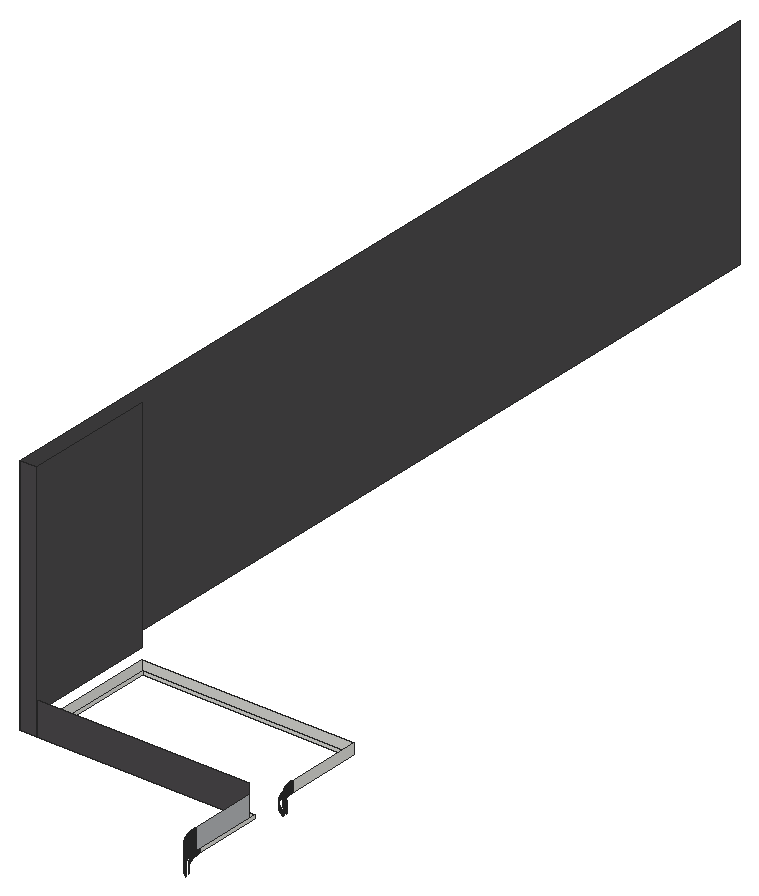
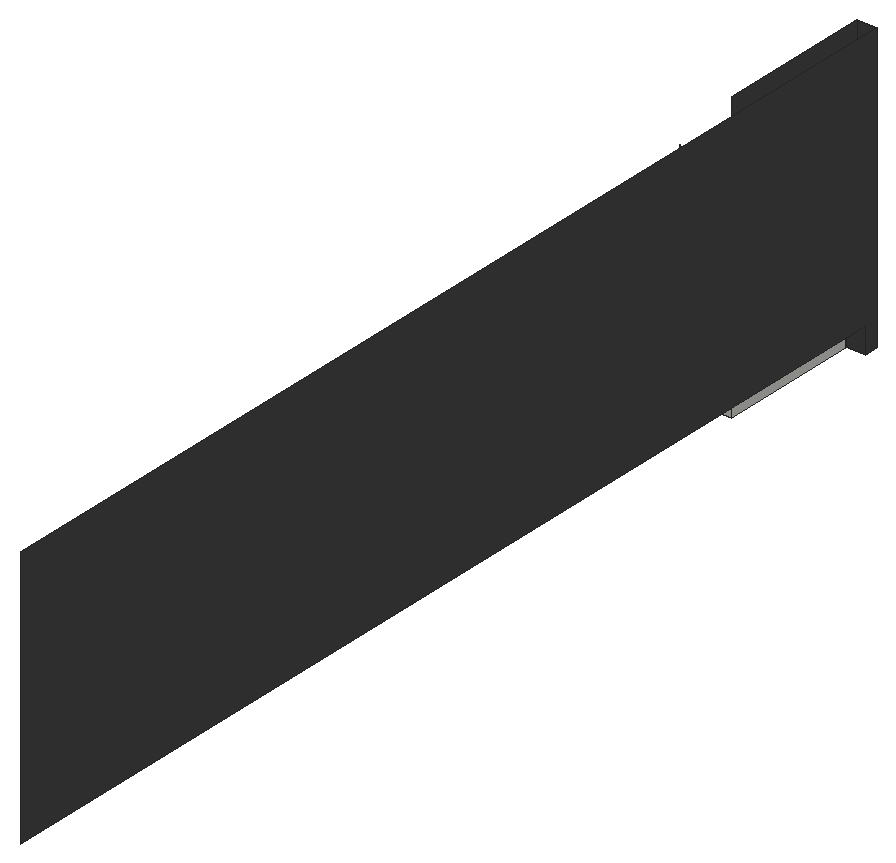
# SketchUp Ruby script. Lengths in inches.
U = 1.inch
M = Sketchup.active_model
def pt(a) = Geom::Point3d.new(a.map { |v| v * U })
def face(e, loops, mat)
  f = e.add_face(loops[0].map { |a| pt(a) })
  loops[1..].each { |l| e.add_face(l.map { |a| pt(a) }).erase! }
  f.material = f.back_material = mat if mat
  f
end
# faces: each face lists its corners as indices into pts; further lists are holes
def faces(e, pts, list, mat = nil) = list.each { |f| face(e, (f[0].is_a?(Array) ? f : [f]).map { |l| l.map { |i| pts[i] } }, mat) }
# xy, xz, yz: faces in a plane at the given z, y or x. An outline is a flat list of corners, or four numbers for a rectangle; further outlines are holes
def ring(l) = l.size == 4 ? [[l[0], l[1]], [l[2], l[1]], [l[2], l[3]], [l[0], l[3]]] : l.each_slice(2).to_a
def flat(e, list, mat, &to3) = list.each { |f| face(e, (f[0].is_a?(Array) ? f : [f]).map { |l| ring(l).map { |u, v| to3.(u, v) } }, mat) }
def xy(e, z, list, mat = nil) = flat(e, list, mat) { |x, y| [x, y, z] }
def xz(e, y, list, mat = nil) = flat(e, list, mat) { |x, z| [x, y, z] }
def yz(e, x, list, mat = nil) = flat(e, list, mat) { |y, z| [x, y, z] }
def lines(e, pts, list) = list.each { |a, b| e.add_line(pt(pts[a]), pt(pts[b])) }
# prism: a flat outline (further loops are holes) pulled along v
def prism(e, loops, v, mat = nil)
  f = face(e, loops, mat); d = Geom::Vector3d.new(v.map { |x| x * U })
  f.pushpull(f.normal.samedirection?(d) ? d.length : -d.length)
end
def box(e, o, s, mat = nil) = prism(e, [[o, [o[0] + s[0], o[1], o[2]], [o[0] + s[0], o[1] + s[1], o[2]], [o[0], o[1] + s[1], o[2]]]], [0, 0, s[2]], mat)
def at(x, y, z, deg = 0) = Geom::Transformation.translation(pt([x, y, z])) * Geom::Transformation.rotation(ORIGIN, Z_AXIS, deg.degrees)
def axes(o, x, y, z) = Geom::Transformation.new([*x, 0, *y, 0, *z, 0, *pt(o).to_a, 1])
def part(name) = M.definitions.add(name)
# library, detail: a bought-in or finely detailed component or shape, given as its bounding box
def library(name, o, s) = part(name).tap { |d| box(d.entities, o, s) }
def detail(e, o, s) = box(e.add_group.entities, o, s)
def put(e, d, t, mat = nil) = e.add_instance(d, t).tap { |i| i.material = mat if mat }
def group(e, t, mat = nil) = e.add_group.tap { |g| g.transformation = t; g.material = mat if mat }.entities
root = M.entities
M.materials.add("1423 AP 8230 BENTONITE").color = [77, 75, 77]
M.materials.add("1427 AP 686 ARMOUR-N").color = [184, 186, 189]
xy(root,114,[[9,180,18,186]],"1423 AP 8230 BENTONITE")
xy(root,114,[[9,180,18,186]],"1427 AP 686 ARMOUR-N")
xz(root,180,[[9,114,18,246],[18,114,134,132]],"1423 AP 8230 BENTONITE")
xz(root,182,[[20,114,136,116]])
xz(root,186,[[9,114,18,126]],"1423 AP 8230 BENTONITE")
xz(root,186,[[9,114,18,120]],"1427 AP 686 ARMOUR-N")
xz(root,250,[[20,114,132,116]])
xz(root,252,[[18,114,134,120]])
yz(root,9,[[180,114,180,246,672,246,672,126,186,126,186,114]],"1423 AP 8230 BENTONITE")
yz(root,18,[[180,114,180,132,186,132,186,120,252,120,252,114]])
yz(root,18,[[180,114,186,114,186,126,252,126,252,246,180,246]],"1423 AP 8230 BENTONITE")
yz(root,20,[[182,114,250,116]])
yz(root,132,[[209.76,114,209.96,116],[209.96,114,210,116],[210,114,250,116]])
yz(root,132.01,[[209.28,114,209.52,116]])
yz(root,134,[[209.78,114,209.97,120],[209.97,114,210,120],[209.97,114,210,120],[210,114,252,120]])
yz(root,134,[[143.6875,114,144,126],[144,114,180,126]],"1427 AP 686 ARMOUR-N")
yz(root,134.01,[[209.35,114,209.57,120]])
yz(root,136,[[143.71,114,144,116],[144,114,182,116]])
p = [[143.89,124.58,126],[143.64,124.77,126],[143.64,124.77,114],[143.89,124.58,114],[143.39,124.96,126],[143.39,124.96,114],
  [143.14,125.15,126],[143.14,125.15,114],[142.9,125.35,126],[142.9,125.35,114],[142.65,125.55,126],[142.65,125.55,114],
  [142.41,125.75,126],[142.41,125.75,114],[142.18,125.96,126],[142.18,125.96,114],[141.94,126.16,126],[141.94,126.16,114],
  [141.71,126.375,126],[141.71,126.375,114],[141.48,126.59,126],[141.48,126.59,114],[141.25,126.81,126],[141.25,126.81,114],
  [141.03,127.03,126],[141.03,127.03,114],[140.81,127.25,126],[140.81,127.25,114],[140.59,127.48,126],[140.59,127.48,114],
  [143.71,127.27,114],[143.49,127.46,114],[143.49,127.46,116],[143.71,127.27,116],[140.375,127.71,126],[140.375,127.71,114],
  [143.28,127.65,114],[143.28,127.65,116],[140.16,127.94,126],[140.16,127.94,114],[143.07,127.84,114],[143.07,127.84,116],
  [142.86,128.04,114],[142.86,128.04,116],[139.96,128.18,126],[139.96,128.18,114],[142.65,128.24,114],[142.65,128.24,116],
  [139.75,128.41,126],[139.75,128.41,114],[142.44,128.44,114],[142.44,128.44,116],[139.55,128.65,126],[139.55,128.65,114],
  [142.24,128.65,114],[142.24,128.65,116],[142.04,128.86,114],[142.04,128.86,116],[139.35,128.9,126],[139.35,128.9,114],
  [139.15,129.14,126],[139.15,129.14,114],[141.84,129.07,114],[141.84,129.07,116],[138.96,129.39,126],[138.96,129.39,114],
  [141.65,129.28,114],[141.65,129.28,116],[141.46,129.49,114],[141.46,129.49,116],[138.77,129.64,126],[138.77,129.64,114],
  [141.27,129.71,114],[141.27,129.71,116],[138.58,129.89,126],[138.58,129.89,114],[141.09,129.93,114],[141.09,129.93,116],
  [138.4,130.15,126],[138.4,130.15,114],[140.9,130.15,114],[140.9,130.15,116],[138.22,130.41,126],[138.22,130.41,114],
  [140.72,130.38,114],[140.72,130.38,116],[138.04,130.67,126],[138.04,130.67,114],[140.55,130.61,114],[140.55,130.61,116],
  [140.37,130.84,114],[140.37,130.84,116],[137.87,130.93,126],[137.87,130.93,114],[140.2,131.07,114],[140.2,131.07,116],
  [137.7,131.19,126],[137.7,131.19,114],[140.03,131.3,114],[140.03,131.3,116],[137.54,131.46,126],[137.54,131.46,114],
  [139.87,131.54,114],[139.87,131.54,116],[137.375,131.73,126],[137.375,131.73,114],[139.71,131.78,114],[139.71,131.78,116],
  [137.22,132,126],[137.22,132,114],[139.55,132.02,114],[139.55,132.02,116],[137.06,132.27,126],[137.06,132.27,114],
  [139.39,132.26,114],[139.39,132.26,116],[136.91,132.55,126],[136.91,132.55,114],[139.24,132.51,114],[139.24,132.51,116],
  [136.76,132.83,126],[136.76,132.83,114],[139.09,132.75,114],[139.09,132.75,116],[136.62,133.1,126],[136.62,133.1,114],
  [138.95,133,114],[138.95,133,116],[138.81,133.25,114],[138.81,133.25,116],[136.48,133.39,126],[136.48,133.39,114],
  [138.67,133.5,114],[138.67,133.5,116],[136.34,133.67,126],[136.34,133.67,114],[138.53,133.76,114],[138.53,133.76,116],
  [136.2,133.95,126],[136.2,133.95,114],[138.4,134.01,114],[138.4,134.01,116],[136.07,134.24,126],[136.07,134.24,114],
  [138.27,134.27,114],[138.27,134.27,116],[135.95,134.53,126],[135.95,134.53,114],[138.14,134.53,114],[138.14,134.53,116],
  [135.83,134.82,126],[135.83,134.82,114],[138.02,134.79,114],[138.02,134.79,116],[135.71,135.11,126],[135.71,135.11,114],
  [137.9,135.05,114],[137.9,135.05,116],[135.59,135.4,126],[135.59,135.4,114],[137.79,135.32,114],[137.79,135.32,116],
  [137.67,135.58,114],[137.67,135.58,116],[135.48,135.69,126],[135.48,135.69,114],[137.57,135.85,114],[137.57,135.85,116],
  [135.375,135.99,126],[135.375,135.99,114],[137.46,136.12,114],[137.46,136.12,116],[135.27,136.29,126],[135.27,136.29,114],
  [137.36,136.39,114],[137.36,136.39,116],[135.17,136.58,126],[135.17,136.58,114],[137.26,136.66,114],[137.26,136.66,116],
  [135.08,136.88,126],[135.08,136.88,114],[137.17,136.93,114],[137.17,136.93,116],[134.99,137.18,126],[134.99,137.18,114],
  [137.08,137.2,114],[137.08,137.2,116],[134.9,137.49,126],[134.9,137.49,114],[136.99,137.48,114],[136.99,137.48,116],
  [134.82,137.79,126],[134.82,137.79,114],[136.91,137.75,114],[136.91,137.75,116],[134.74,138.09,126],[134.74,138.09,114],
  [136.83,138.03,114],[136.83,138.03,116],[136.75,138.31,114],[136.75,138.31,116],[134.66,138.4,126],[134.66,138.4,114],
  [136.68,138.58,114],[136.68,138.58,116],[134.59,138.7,126],[134.59,138.7,114],[136.61,138.86,114],[136.61,138.86,116],
  [134.52,139.01,126],[134.52,139.01,114],[136.54,139.14,114],[136.54,139.14,116],[134.46,139.32,126],[134.46,139.32,114],
  [136.48,139.43,114],[136.48,139.43,116],[134.4,139.625,126],[134.4,139.625,114],[136.42,139.71,114],[136.42,139.71,116],
  [134.35,139.9375,126],[134.35,139.9375,114],[136.37,139.99,114],[136.37,139.99,116],[134.3,140.25,126],[134.3,140.25,114],
  [136.32,140.27,114],[136.32,140.27,116],[134.25,140.56,126],[134.25,140.56,114],[136.27,140.56,114],[136.27,140.56,116],
  [134.21,140.87,126],[134.21,140.87,114],[136.23,140.84,114],[136.23,140.84,116],[136.1875,141.13,114],[136.1875,141.13,116],
  [134.17,141.18,126],[134.17,141.18,114],[136.15,141.41,114],[136.15,141.41,116],[134.13,141.49,126],[134.13,141.49,114],
  [136.12,141.7,114],[136.12,141.7,116],[134.1,141.8,126],[134.1,141.8,114],[136.09,141.99,114],[136.09,141.99,116],
  [134.07,142.12,126],[134.07,142.12,114],[136.07,142.27,114],[136.07,142.27,116],[134.05,142.43,126],[134.05,142.43,114],
  [136.05,142.5625,114],[136.05,142.5625,116],[134.03,142.74,126],[134.03,142.74,114],[136.03,142.85,114],[136.03,142.85,116],
  [134.02,143.06,126],[134.02,143.06,114],[136.02,143.14,114],[136.02,143.14,116],[134.01,143.37,126],[134.01,143.37,114],
  [136.01,143.42,114],[136.01,143.42,116],[134,143.6875,126],[134,143.6875,114],[136,143.71,114],[136,143.71,116],
  [143.57,191.86,114],[143.79,191.76,114],[143.79,191.76,116],[143.57,191.86,116],[143.35,191.97,114],[143.35,191.97,116],
  [143.14,192.07,114],[143.14,192.07,116],[142.92,192.18,114],[142.92,192.18,116],[142.71,192.29,114],[142.71,192.29,116],
  [142.49,192.4,114],[142.49,192.4,116],[142.28,192.52,114],[142.28,192.52,116],[142.07,192.64,114],[142.07,192.64,116],
  [141.86,192.76,114],[141.86,192.76,116],[141.65,192.88,114],[141.65,192.88,116],[141.45,193.01,114],[141.45,193.01,116],
  [141.24,193.14,114],[141.24,193.14,116],[141.04,193.27,114],[141.04,193.27,116],[140.84,193.4,114],[140.84,193.4,116],
  [140.64,193.54,114],[140.64,193.54,116],[140.44,193.68,114],[140.44,193.68,116],[140.24,193.82,114],[140.24,193.82,116],
  [140.05,193.96,114],[140.05,193.96,116],[139.86,194.11,114],[139.86,194.11,116],[143.63,194.0625,120],[143.83,193.96,120],
  [143.83,193.96,114],[143.63,194.0625,114],[139.67,194.26,114],[139.67,194.26,116],[143.44,194.16,120],[143.44,194.16,114],
  [143.25,194.27,120],[143.25,194.27,114],[139.48,194.41,114],[139.48,194.41,116],[143.0625,194.375,120],[143.0625,194.375,114],
  [139.29,194.56,114],[139.29,194.56,116],[142.875,194.48,120],[142.875,194.48,114],[142.6875,194.6,120],[142.6875,194.6,114],
  [139.1,194.71,114],[139.1,194.71,116],[142.5,194.71,120],[142.5,194.71,114],[138.92,194.87,114],[138.92,194.87,116],
  [142.32,194.83,120],[142.32,194.83,114],[142.14,194.94,120],[142.14,194.94,114],[138.74,195.03,114],[138.74,195.03,116],
  [141.95,195.0625,120],[141.95,195.0625,114],[138.56,195.19,114],[138.56,195.19,116],[141.77,195.1875,120],[141.77,195.1875,114],
  [138.38,195.35,114],[138.38,195.35,116],[141.6,195.3125,120],[141.6,195.3125,114],[141.42,195.4375,120],[141.42,195.4375,114],
  [138.2,195.52,114],[138.2,195.52,116],[141.24,195.57,120],[141.24,195.57,114],[138.03,195.6875,114],[138.03,195.6875,116],
  [141.07,195.7,120],[141.07,195.7,114],[137.86,195.86,114],[137.86,195.86,116],[140.9,195.83,120],[140.9,195.83,114],
  [140.73,195.97,120],[140.73,195.97,114],[137.6875,196.03,114],[137.6875,196.03,116],[137.52,196.2,114],[137.52,196.2,116],
  [140.56,196.1,120],[140.56,196.1,114],[140.39,196.24,120],[140.39,196.24,114],[137.35,196.38,114],[137.35,196.38,116],
  [140.23,196.38,120],[140.23,196.38,114],[137.19,196.56,114],[137.19,196.56,116],[140.0625,196.53,120],[140.0625,196.53,114],
  [139.9,196.67,120],[139.9,196.67,114],[137.03,196.74,114],[137.03,196.74,116],[136.87,196.92,114],[136.87,196.92,116],
  [139.74,196.82,120],[139.74,196.82,114],[139.58,196.97,120],[139.58,196.97,114],[136.71,197.1,114],[136.71,197.1,116],
  [139.43,197.12,120],[139.43,197.12,114],[136.56,197.29,114],[136.56,197.29,116],[139.27,197.27,120],[139.27,197.27,114],
  [136.41,197.48,114],[136.41,197.48,116],[139.12,197.43,120],[139.12,197.43,114],[138.97,197.58,120],[138.97,197.58,114],
  [136.26,197.67,114],[136.26,197.67,116],[138.82,197.74,120],[138.82,197.74,114],[136.11,197.86,114],[136.11,197.86,116],
  [138.67,197.9,120],[138.67,197.9,114],[135.96,198.05,114],[135.96,198.05,116],[138.53,198.0625,120],[138.53,198.0625,114],
  [135.82,198.24,114],[135.82,198.24,116],[138.38,198.23,120],[138.38,198.23,114],[135.68,198.44,114],[135.68,198.44,116],
  [138.24,198.39,120],[138.24,198.39,114],[135.54,198.64,114],[135.54,198.64,116],[138.1,198.56,120],[138.1,198.56,114],
  [135.4,198.84,114],[135.4,198.84,116],[137.97,198.73,120],[137.97,198.73,114],[137.83,198.9,120],[137.83,198.9,114],
  [135.27,199.04,114],[135.27,199.04,116],[137.7,199.07,120],[137.7,199.07,114],[135.14,199.24,114],[135.14,199.24,116],
  [137.57,199.24,120],[137.57,199.24,114],[135.01,199.45,114],[135.01,199.45,116],[137.4375,199.42,120],[137.4375,199.42,114],
  [134.88,199.65,114],[134.88,199.65,116],[137.3125,199.6,120],[137.3125,199.6,114],[137.1875,199.77,120],[137.1875,199.77,114],
  [134.76,199.86,114],[134.76,199.86,116],[137.0625,199.95,120],[137.0625,199.95,114],[134.64,200.07,114],[134.64,200.07,116],
  [136.94,200.14,120],[136.94,200.14,114],[134.52,200.28,114],[134.52,200.28,116],[136.83,200.32,120],[136.83,200.32,114],
  [134.4,200.49,114],[134.4,200.49,116],[136.71,200.5,120],[136.71,200.5,114],[134.29,200.71,114],[134.29,200.71,116],
  [136.6,200.6875,120],[136.6,200.6875,114],[134.18,200.92,114],[134.18,200.92,116],[136.48,200.875,120],[136.48,200.875,114],
  [134.07,201.14,114],[134.07,201.14,116],[136.375,201.0625,120],[136.375,201.0625,114],[133.97,201.35,114],[133.97,201.35,116],
  [136.27,201.25,120],[136.27,201.25,114],[136.16,201.44,120],[136.16,201.44,114],[133.86,201.57,114],[133.86,201.57,116],
  [136.0625,201.63,120],[136.0625,201.63,114],[133.76,201.79,114],[133.76,201.79,116],[135.96,201.83,120],[135.96,201.83,114],
  [133.66,202.01,114],[133.66,202.01,116],[135.86,202.02,120],[135.86,202.02,114],[133.57,202.23,114],[133.57,202.23,116],
  [135.77,202.22,120],[135.77,202.22,114],[133.48,202.46,114],[133.48,202.46,116],[135.68,202.41,120],[135.68,202.41,114],
  [135.59,202.61,120],[135.59,202.61,114],[133.39,202.68,114],[133.39,202.68,116],[135.5,202.8125,120],[135.5,202.8125,114],
  [133.3,202.91,114],[133.3,202.91,116],[135.41,203.01,120],[135.41,203.01,114],[133.22,203.13,114],[133.22,203.13,116],
  [135.33,203.21,120],[135.33,203.21,114],[133.13,203.36,114],[133.13,203.36,116],[135.25,203.41,120],[135.25,203.41,114],
  [133.05,203.59,114],[133.05,203.59,116],[135.17,203.62,120],[135.17,203.62,114],[132.98,203.82,114],[132.98,203.82,116],
  [135.09,203.82,120],[135.09,203.82,114],[132.91,204.05,114],[132.91,204.05,116],[135.02,204.03,120],[135.02,204.03,114],
  [132.84,204.28,114],[132.84,204.28,116],[134.95,204.23,120],[134.95,204.23,114],[134.88,204.4375,120],[134.88,204.4375,114],
  [132.77,204.51,114],[132.77,204.51,116],[134.82,204.64,120],[134.82,204.64,114],[132.7,204.75,114],[132.7,204.75,116],
  [134.75,204.85,120],[134.75,204.85,114],[132.64,204.98,114],[132.64,204.98,116],[134.69,205.0625,120],[134.69,205.0625,114],
  [132.58,205.21,114],[132.58,205.21,116],[134.63,205.27,120],[134.63,205.27,114],[132.52,205.45,114],[132.52,205.45,116],
  [134.58,205.48,120],[134.58,205.48,114],[132.47,205.68,114],[132.47,205.68,116],[134.52,205.69,120],[134.52,205.69,114],
  [132.42,205.92,114],[132.42,205.92,116],[134.47,205.9,120],[134.47,205.9,114],[132.37,206.16,114],[132.37,206.16,116],
  [134.42,206.12,120],[134.42,206.12,114],[134.38,206.33,120],[134.38,206.33,114],[132.33,206.39,114],[132.33,206.39,116],
  [134.34,206.54,120],[134.34,206.54,114],[132.29,206.63,114],[132.29,206.63,116],[134.29,206.76,120],[134.29,206.76,114],
  [132.25,206.87,114],[132.25,206.87,116],[134.26,206.97,120],[134.26,206.97,114],[132.21,207.11,114],[132.21,207.11,116],
  [134.22,207.18,120],[134.22,207.18,114],[132.18,207.35,114],[132.18,207.35,116],[134.1875,207.4,120],[134.1875,207.4,114],
  [132.15,207.59,114],[132.15,207.59,116],[134.16,207.61,120],[134.16,207.61,114],[132.12,207.83,114],[132.12,207.83,116],
  [134.13,207.83,120],[134.13,207.83,114],[132.09,208.07,114],[132.09,208.07,116],[134.11,208.05,120],[134.11,208.05,114],
  [134.08,208.26,120],[134.08,208.26,114],[132.07,208.31,114],[132.07,208.31,116],[132.05,208.55,114],[132.05,208.55,116],
  [134.0625,208.48,120],[134.0625,208.48,114],[134.05,208.7,120],[134.05,208.7,114],[132.04,208.79,114],[132.04,208.79,116],
  [134.03,208.91,120],[134.03,208.91,114],[132.02,209.03,114],[132.02,209.03,116],[134.02,209.13,120],[134.02,209.13,114],
  [132.01,209.28,114],[132.01,209.28,116],[134.01,209.35,120],[134.01,209.35,114],[132,209.76,114],[132.01,209.52,114],
  [132.01,209.52,116],[132,209.76,116],[134,209.78,120],[134.01,209.57,120],[134.01,209.57,114],[134,209.78,114]]
faces(root,p,[[0,1,2,3],[1,4,5,2],[4,6,7,5],[6,8,9,7],[8,10,11,9],[10,12,13,11],[12,14,15,13],[14,16,17,15],
  [16,18,19,17],[18,20,21,19],[20,22,23,21],[22,24,25,23],[24,26,27,25],[26,28,29,27],[28,34,35,29],[34,38,39,35],
  [38,44,45,39],[44,48,49,45],[48,52,53,49],[52,58,59,53],[58,60,61,59],[60,64,65,61],[64,70,71,65],[70,74,75,71],
  [74,78,79,75],[78,82,83,79],[82,86,87,83],[86,92,93,87],[92,96,97,93],[96,100,101,97],[100,104,105,101],[104,108,109,105],
  [108,112,113,109],[112,116,117,113],[116,120,121,117],[120,124,125,121],[124,130,131,125],[130,134,135,131],[134,138,139,135],[138,142,143,139],
  [142,146,147,143],[146,150,151,147],[150,154,155,151],[154,158,159,155],[158,164,165,159],[164,168,169,165],[168,172,173,169],[172,176,177,173],
  [176,180,181,177],[180,184,185,181],[184,188,189,185],[188,192,193,189],[192,196,197,193],[196,202,203,197],[202,206,207,203],[206,210,211,207],
  [210,214,215,211],[214,218,219,215],[218,222,223,219],[222,226,227,223],[226,230,231,227],[230,234,235,231],[234,240,241,235],[240,244,245,241],
  [244,248,249,245],[248,252,253,249],[252,256,257,253],[256,260,261,257],[260,264,265,261],[264,268,269,265],[268,272,273,269]],"1427 AP 686 ARMOUR-N")
faces(root,p,[[30,31,32,33],[31,36,37,32],[36,40,41,37],[40,42,43,41],[42,46,47,43],[46,50,51,47],[50,54,55,51],[54,56,57,55],
  [56,62,63,57],[62,66,67,63],[66,68,69,67],[68,72,73,69],[72,76,77,73],[76,80,81,77],[80,84,85,81],[84,88,89,85],
  [88,90,91,89],[90,94,95,91],[94,98,99,95],[98,102,103,99],[102,106,107,103],[106,110,111,107],[110,114,115,111],[114,118,119,115],
  [118,122,123,119],[122,126,127,123],[126,128,129,127],[128,132,133,129],[132,136,137,133],[136,140,141,137],[140,144,145,141],[144,148,149,145],
  [148,152,153,149],[152,156,157,153],[156,160,161,157],[160,162,163,161],[162,166,167,163],[166,170,171,167],[170,174,175,171],[174,178,179,175],
  [178,182,183,179],[182,186,187,183],[186,190,191,187],[190,194,195,191],[194,198,199,195],[198,200,201,199],[200,204,205,201],[204,208,209,205],
  [208,212,213,209],[212,216,217,213],[216,220,221,217],[220,224,225,221],[224,228,229,225],[228,232,233,229],[232,236,237,233],[236,238,239,237],
  [238,242,243,239],[242,246,247,243],[246,250,251,247],[250,254,255,251],[254,258,259,255],[258,262,263,259],[262,266,267,263],[266,270,271,267],
  [270,274,275,271],[276,277,278,279],[280,276,279,281],[282,280,281,283],[284,282,283,285],[286,284,285,287],[288,286,287,289],[290,288,289,291],
  [292,290,291,293],[294,292,293,295],[296,294,295,297],[298,296,297,299],[300,298,299,301],[302,300,301,303],[304,302,303,305],[306,304,305,307],
  [308,306,307,309],[310,308,309,311],[312,310,311,313],[314,312,313,315],[316,317,318,319],[320,314,315,321],[322,316,319,323],[324,322,323,325],
  [326,320,321,327],[328,324,325,329],[330,326,327,331],[332,328,329,333],[334,332,333,335],[336,330,331,337],[338,334,335,339],[340,336,337,341],
  [342,338,339,343],[344,342,343,345],[346,340,341,347],[348,344,345,349],[350,346,347,351],[352,348,349,353],[354,350,351,355],[356,352,353,357],
  [358,356,357,359],[360,354,355,361],[362,358,359,363],[364,360,361,365],[366,362,363,367],[368,364,365,369],[370,366,367,371],[372,370,371,373],
  [374,368,369,375],[376,374,375,377],[378,372,373,379],[380,378,379,381],[382,376,377,383],[384,380,381,385],[386,382,383,387],[388,384,385,389],
  [390,388,389,391],[392,386,387,393],[394,392,393,395],[396,390,391,397],[398,396,397,399],[400,394,395,401],[402,398,399,403],[404,400,401,405],
  [406,402,403,407],[408,404,405,409],[410,406,407,411],[412,410,411,413],[414,408,409,415],[416,412,413,417],[418,414,415,419],[420,416,417,421],
  [422,418,419,423],[424,420,421,425],[426,422,423,427],[428,424,425,429],[430,426,427,431],[432,428,429,433],[434,430,431,435],[436,432,433,437],
  [438,434,435,439],[440,436,437,441],[442,440,441,443],[444,438,439,445],[446,442,443,447],[448,444,445,449],[450,446,447,451],[452,448,449,453],
  [454,450,451,455],[456,452,453,457],[458,454,455,459],[460,458,459,461],[462,456,457,463],[464,460,461,465],[466,462,463,467],[468,464,465,469],
  [470,466,467,471],[472,468,469,473],[474,470,471,475],[476,472,473,477],[478,474,475,479],[480,476,477,481],[482,478,479,483],[484,480,481,485],
  [486,482,483,487],[488,484,485,489],[490,486,487,491],[492,488,489,493],[494,492,493,495],[496,490,491,497],[498,494,495,499],[500,496,497,501],
  [502,498,499,503],[504,500,501,505],[506,502,503,507],[508,504,505,509],[510,506,507,511],[512,508,509,513],[514,510,511,515],[516,514,515,517],
  [518,512,513,519],[520,516,517,521],[522,518,519,523],[524,520,521,525],[526,522,523,527],[528,524,525,529],[530,526,527,531],[532,528,529,533],
  [534,530,531,535],[536,532,533,537],[538,534,535,539],[540,536,537,541],[542,538,539,543],[544,540,541,545],[546,542,543,547],[548,544,545,549],
  [550,548,549,551],[552,546,547,553],[554,550,551,555],[556,552,553,557],[558,554,555,559],[560,556,557,561],[562,558,559,563],[564,560,561,565],
  [566,562,563,567],[568,564,565,569],[570,566,567,571],[572,568,569,573],[574,570,571,575],[576,572,573,577],[578,574,575,579],[580,576,577,581],
  [582,578,579,583],[584,582,583,585],[586,580,581,587],[588,584,585,589],[590,586,587,591],[592,588,589,593],[594,590,591,595],[596,592,593,597],
  [598,594,595,599],[600,596,597,601],[602,598,599,603],[604,600,601,605],[606,602,603,607],[608,604,605,609],[610,606,607,611],[612,608,609,613],
  [614,610,611,615],[616,612,613,617],[618,616,617,619],[620,614,615,621],[622,620,621,623],[624,618,619,625],[626,624,625,627],[628,622,623,629],
  [630,626,627,631],[632,628,629,633],[634,630,631,635],[636,632,633,637],[638,634,635,639],[640,641,642,643],[644,645,646,647]])
